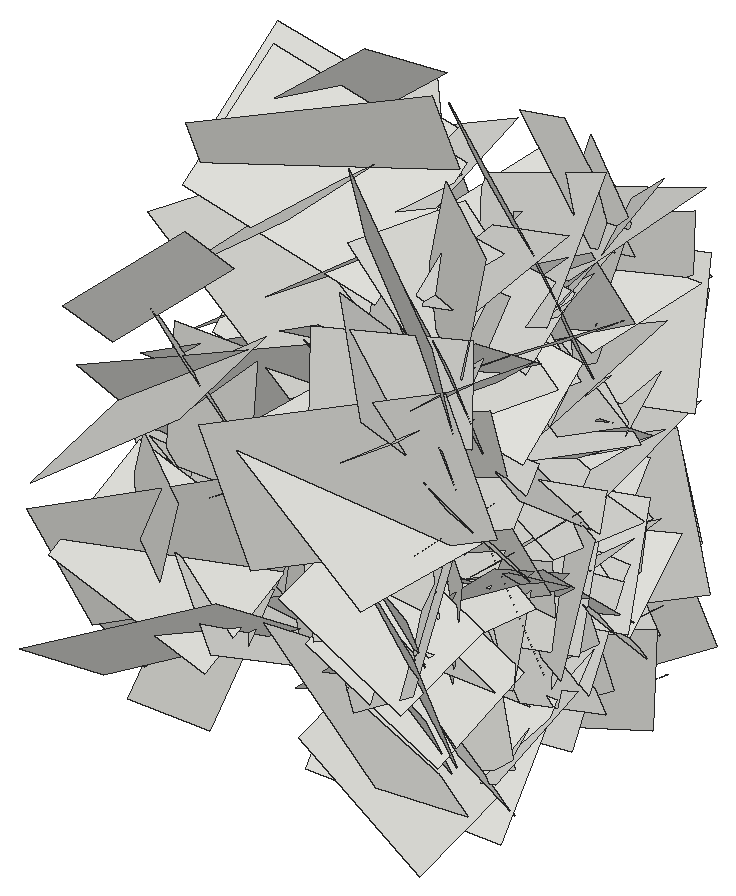
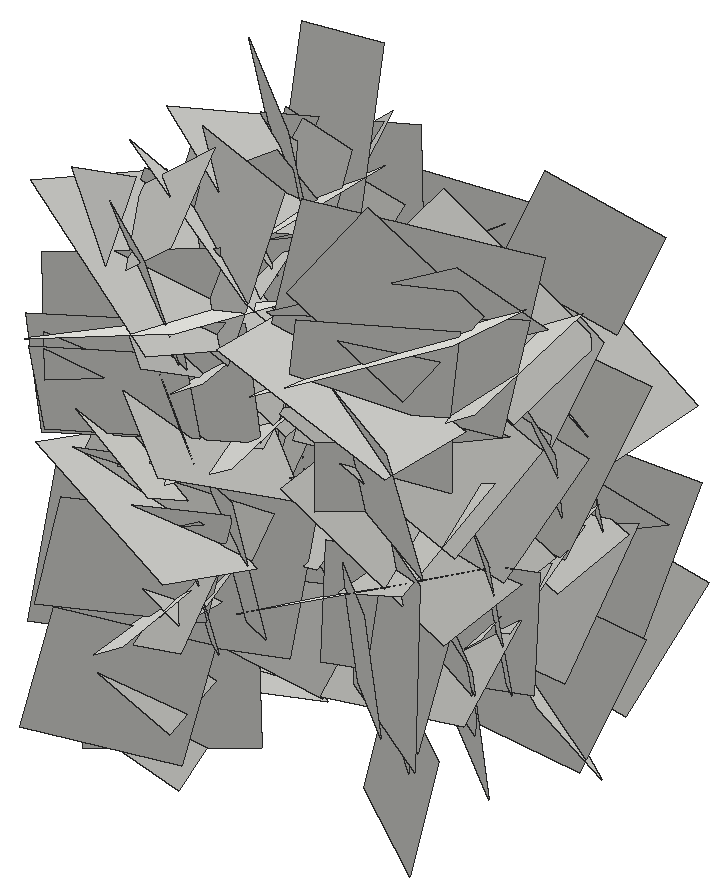
# SketchUp Ruby script. Lengths in inches.
U = 1.inch
M = Sketchup.active_model
def pt(a) = Geom::Point3d.new(a.map { |v| v * U })
def face(e, loops, mat)
  f = e.add_face(loops[0].map { |a| pt(a) })
  loops[1..].each { |l| e.add_face(l.map { |a| pt(a) }).erase! }
  f.material = f.back_material = mat if mat
  f
end
# faces: each face lists its corners as indices into pts; further lists are holes
def faces(e, pts, list, mat = nil) = list.each { |f| face(e, (f[0].is_a?(Array) ? f : [f]).map { |l| l.map { |i| pts[i] } }, mat) }
# xy, xz, yz: faces in a plane at the given z, y or x. An outline is a flat list of corners, or four numbers for a rectangle; further outlines are holes
def ring(l) = l.size == 4 ? [[l[0], l[1]], [l[2], l[1]], [l[2], l[3]], [l[0], l[3]]] : l.each_slice(2).to_a
def flat(e, list, mat, &to3) = list.each { |f| face(e, (f[0].is_a?(Array) ? f : [f]).map { |l| ring(l).map { |u, v| to3.(u, v) } }, mat) }
def xy(e, z, list, mat = nil) = flat(e, list, mat) { |x, y| [x, y, z] }
def xz(e, y, list, mat = nil) = flat(e, list, mat) { |x, z| [x, y, z] }
def yz(e, x, list, mat = nil) = flat(e, list, mat) { |y, z| [x, y, z] }
def lines(e, pts, list) = list.each { |a, b| e.add_line(pt(pts[a]), pt(pts[b])) }
# prism: a flat outline (further loops are holes) pulled along v
def prism(e, loops, v, mat = nil)
  f = face(e, loops, mat); d = Geom::Vector3d.new(v.map { |x| x * U })
  f.pushpull(f.normal.samedirection?(d) ? d.length : -d.length)
end
def box(e, o, s, mat = nil) = prism(e, [[o, [o[0] + s[0], o[1], o[2]], [o[0] + s[0], o[1] + s[1], o[2]], [o[0], o[1] + s[1], o[2]]]], [0, 0, s[2]], mat)
def at(x, y, z, deg = 0) = Geom::Transformation.translation(pt([x, y, z])) * Geom::Transformation.rotation(ORIGIN, Z_AXIS, deg.degrees)
def axes(o, x, y, z) = Geom::Transformation.new([*x, 0, *y, 0, *z, 0, *pt(o).to_a, 1])
def part(name) = M.definitions.add(name)
# library, detail: a bought-in or finely detailed component or shape, given as its bounding box
def library(name, o, s) = part(name).tap { |d| box(d.entities, o, s) }
def detail(e, o, s) = box(e.add_group.entities, o, s)
def put(e, d, t, mat = nil) = e.add_instance(d, t).tap { |i| i.material = mat if mat }
def group(e, t, mat = nil) = e.add_group.tap { |g| g.transformation = t; g.material = mat if mat }.entities
root = M.entities
c1 = part("Component\#6")
p = [[0.01,0,0],[0,3.24,4.54],[4.32,3.24,4.54],[4.33,0,0]]
faces(c1.entities,p,[[0,1,2,3]])
put(root,c1,axes([414.68,149.09,36.34],[0.1737,0.35213,-1.24285],[-0.08,-1.24806,-0.36356],[-1.36694,0.11779,-0.13666]))
put(root,c1,axes([400.91,150.86,30.47],[0.14962,-1.13409,-0.09371],[-0.03493,-0.09847,1.14197],[1.20573,0.13788,0.04471]))
put(root,c1,axes([414.68,150.86,30.47],[-0.14962,-1.13409,-0.09371],[0.03493,-0.09847,1.14197],[-1.20573,0.13788,0.04471]))
put(root,c1,axes([414.68,150.98,27.43],[-0.11329,-0.77541,-0.3635],[0.07754,-0.37325,0.77469],[-0.90445,0.06513,0.11195]))
put(root,c1,axes([410.71,147.9,27.03],[-0.12769,0.03013,0.63893],[-0.01482,0.64988,-0.03329],[0.67785,0.01989,0.11963]))
put(root,c1,axes([404.88,147.9,27.03],[0.12769,0.03013,0.63893],[0.01482,0.64988,-0.03329],[-0.67785,0.01989,0.11963]))
put(root,c1,axes([404.88,149.08,38.35],[-0.0057,0.54335,-0.52891],[0.23788,-0.50408,-0.52014],[-0.76776,-0.16022,-0.15723]))
put(root,c1,axes([410.71,149.08,38.35],[0.0057,0.54335,-0.52891],[-0.23788,-0.50408,-0.52014],[0.76776,-0.16022,-0.15723]))
put(root,c1,axes([400.91,150.2,21.48],[0.03659,-0.96074,0.6365],[0.08804,0.6372,0.9573],[1.21843,-0.01719,-0.08829]))
put(root,c1,axes([414.68,150.2,21.48],[-0.03659,-0.96074,0.6365],[-0.08804,0.6372,0.9573],[-1.21843,-0.01719,-0.08829]))
put(root,c1,axes([414.68,150.44,37.52],[0.01758,-0.03984,-0.83316],[-0.08726,-0.82933,0.03802],[-0.87984,0.08145,-0.02042]))
put(root,c1,axes([410.71,150.81,32.67],[-0.03105,-0.70657,0.01303],[0.00041,0.01303,0.70717],[0.74909,-0.02929,0.00015]))
put(root,c1,axes([410.71,149.71,29.1],[0.04042,0.22115,-0.567],[0.10046,-0.56334,-0.21335],[0.63725,0.07479,0.0696]))
put(root,c1,axes([410.71,147.16,24.1],[-0.03025,0.92414,0.23442],[-0.23339,0.2218,-0.90118],[0.98329,0.08108,-0.20669]))
put(root,c1,axes([410.71,149.63,26.39],[-0.05575,0.3601,-0.58557],[0.15834,-0.56726,-0.36226],[0.71127,0.15451,0.03475]))
put(root,c1,axes([400.91,147.58,26.68],[0.22766,0.71104,0.67114],[-0.02672,0.69094,-0.72395],[1.03608,-0.13842,-0.16614]))
put(root,c1,axes([414.68,147.58,26.68],[-0.22766,0.71104,0.67114],[0.02672,0.69094,-0.72395],[-1.03608,-0.13842,-0.16614]))
put(root,c1,axes([400.91,149.67,23.37],[-0.09539,-0.59855,1.14231],[0.08783,1.14003,0.60389],[1.36418,-0.11525,0.041]))
put(root,c1,axes([414.68,149.67,23.37],[0.09539,-0.59855,1.14231],[-0.08783,1.14003,0.60389],[-1.36418,-0.11525,0.041]))
put(root,c1,axes([414.68,149.65,34.23],[0.2234,-0.54463,1.08834],[0.02633,1.10624,0.54877],[-1.28976,-0.07175,0.19972]))
put(root,c1,axes([410.71,151.89,27.92],[0.07457,-0.37507,-0.49968],[-0.035,-0.50437,0.37394],[0.66135,0.0156,0.07613]))
put(root,c1,axes([414.68,152.86,25.21],[-0.07237,-0.84668,-0.40971],[0.16913,-0.41526,0.83156],[-0.98259,-0.00911,0.17331]))
put(root,c1,axes([410.71,153.18,27.99],[-0.08911,-1.01671,-0.11332],[-0.1646,-0.0997,1.00972],[1.07181,-0.09984,0.14565]))
put(root,c1,axes([414.68,150.4,30.92],[-0.04252,-0.27759,0.76161],[-0.13298,0.75548,0.26875],[-0.84891,-0.10444,-0.08025]))
put(root,c1,axes([400.91,151.25,34.8],[0.16779,0.3958,-0.75565],[0.05631,-0.77163,-0.39305],[0.90246,-0.02545,0.16502]))
put(root,c1,axes([414.68,151.25,34.8],[-0.16779,0.3958,-0.75565],[-0.05631,-0.77163,-0.39305],[-0.90246,-0.02545,0.16502]))
put(root,c1,axes([410.71,152.86,32.22],[-0.07765,-0.95123,0.12327],[-0.10469,0.13045,0.94796],[1.01133,-0.05954,0.1076]))
put(root,c1,axes([414.68,150.92,33.45],[0.01124,-0.40239,0.85237],[-0.02564,0.85203,0.40253],[-0.99881,-0.0264,-0.00074]))
put(root,c1,axes([414.68,150.56,37.37],[-0.01495,0.72639,-0.4873],[-0.06872,-0.48689,-0.7239],[-0.92463,0.02444,0.06168]))
put(root,c1,axes([410.71,150.69,21.46],[-0.08617,-0.06424,0.73191],[0.1147,0.7273,0.07585],[0.77031,-0.11548,0.07058]))
put(root,c1,axes([400.91,154.4,23.625],[-0.0407,-0.65785,-0.83395],[0.03781,-0.83482,0.65689],[1.12528,0.00426,-0.05223]))
put(root,c1,axes([414.68,154.4,23.625],[0.0407,-0.65785,-0.83395],[-0.03781,-0.83482,0.65689],[-1.12528,0.00426,-0.05223]))
put(root,c1,axes([400.91,153.43,27.14],[0.15407,-0.97446,-0.01303],[0.08051,-0.00181,0.98239],[1.02988,0.14592,-0.07485]))
put(root,c1,axes([414.68,153.43,27.14],[-0.15407,-0.97446,-0.01303],[-0.08051,-0.00181,0.98239],[-1.02988,0.14592,-0.07485]))
put(root,c1,axes([400.91,153.58,31.99],[0.17505,-0.32324,-0.90395],[0.10086,-0.9072,0.34179],[1.0126,0.14624,0.12223]))
put(root,c1,axes([414.68,153.58,31.99],[-0.17505,-0.32324,-0.90395],[-0.10086,-0.9072,0.34179],[-1.0126,0.14624,0.12223]))
put(root,c1,axes([410.71,152.7,33.94],[-0.15183,0.13661,-0.74127],[0.04087,-0.75222,-0.14607],[0.79793,0.06452,-0.13357]))
put(root,c1,axes([410.71,153.52,29.46],[-0.08102,0.00764,-0.81457],[-0.10707,-0.81193,0.00187],[0.85682,-0.10074,-0.07679]))
put(root,c1,axes([400.91,152.42,20.54],[-0.05004,-0.6691,0.77955],[0.05919,0.77755,0.67076],[1.08735,-0.07312,-0.00064]))
put(root,c1,axes([414.68,152.42,20.54],[0.05004,-0.6691,0.77955],[-0.05919,0.77755,0.67076],[-1.08735,-0.07312,-0.00064]))
put(root,c1,axes([410.71,154.14,39.875],[-0.07687,-0.17009,-0.90128],[-0.07958,-0.89996,0.17589],[0.96896,-0.0874,-0.05706]))
put(root,c1,axes([414.68,152.27,30.34],[-0.04267,0.47891,-0.74389],[-0.05776,-0.74459,-0.47642],[-0.93603,0.02411,0.06331]))
put(root,c1,axes([400.91,153.125,28.17],[-0.03085,-0.9293,0.97672],[0.26234,0.95667,0.91759],[1.40479,-0.19906,-0.14991]))
put(root,c1,axes([414.68,153.125,28.17],[0.03085,-0.9293,0.97672],[-0.26234,0.95667,0.91759],[-1.40479,-0.19906,-0.14991]))
put(root,c1,axes([400.91,153.14,23.91],[0.18,-1.08552,0.79109],[0.08355,0.80406,1.08641],[1.42134,0.0902,-0.16405]))
put(root,c1,axes([414.68,153.14,23.91],[-0.18,-1.08552,0.79109],[-0.08355,0.80406,1.08641],[-1.42134,0.0902,-0.16405]))
put(root,c1,axes([400.91,151.45,29.33],[0.11063,1.17252,-0.59491],[-0.28501,-0.56514,-1.16101],[1.36425,-0.21315,-0.19431]))
put(root,c1,axes([414.68,151.45,29.33],[-0.11063,1.17252,-0.59491],[0.28501,-0.56514,-1.16101],[-1.36425,-0.21315,-0.19431]))
put(root,c1,axes([410.71,155.3,36.05],[-0.02231,-0.46484,-0.62566],[-0.10069,-0.6197,0.4636],[0.82005,-0.08874,0.0399]))
put(root,c1,axes([400.91,152.14,28.92],[0.00837,0.82237,-0.50147],[0.16225,-0.49618,-0.8113],[1.00803,0.07304,0.13474]))
put(root,c1,axes([414.68,152.14,28.92],[-0.00837,0.82237,-0.50147],[-0.16225,-0.49618,-0.8113],[-1.00803,0.07304,0.13474]))
put(root,c1,axes([414.68,155.63,34.51],[0.04715,-0.7148,-0.47013],[-0.06325,-0.47221,0.71232],[-0.90467,-0.00424,-0.0743]))
put(root,c1,axes([414.68,151.43,29.49],[0.01376,0.93036,0.01045],[0.09599,0.00914,-0.92605],[-0.98156,0.01394,-0.09041]))
put(root,c1,axes([400.91,155.57,33.875],[0.13701,-1.11756,0.11199],[-0.07264,0.10468,1.12363],[1.18833,0.13525,0.05577]))
put(root,c1,axes([414.68,155.57,33.875],[-0.13701,-1.11756,0.11199],[0.07264,0.10468,1.12363],[-1.18833,0.13525,0.05577]))
put(root,c1,axes([410.71,156.34,37.48],[-0.20366,-0.78098,-0.33642],[0.07649,-0.35863,0.79133],[0.89812,-0.14656,-0.14368]))
put(root,c1,axes([414.68,152.31,24.83],[-0.14132,0.38772,0.61473],[-0.11706,0.60692,-0.40674],[-0.76145,-0.16526,-0.05156]))
put(root,c1,axes([410.71,152.23,36.27],[0.17612,0.33723,0.58016],[-0.03508,0.60107,-0.33991],[0.71045,-0.05392,-0.16061]))
put(root,c1,axes([414.68,151.53,22],[0.08087,0.78957,0.40941],[-0.10212,0.41583,-0.78401],[-0.93722,0.02282,0.12075]))
put(root,c1,axes([400.91,156.79,29.67],[0.01777,-0.29003,-1.18393],[-0.05362,-1.18318,0.28913],[1.29096,-0.04516,0.0283]))
put(root,c1,axes([414.68,156.79,29.67],[-0.01777,-0.29003,-1.18393],[0.05362,-1.18318,0.28913],[-1.29096,-0.04516,0.0283]))
put(root,c1,axes([410.71,153.82,25.23],[0.04726,-0.11023,0.59197],[0.093,0.58845,0.10297],[0.63147,-0.07841,-0.05947]))
put(root,c1,axes([410.71,156.05,22.34],[0.04217,-0.56806,-0.37659],[0.07293,-0.37196,0.56834],[0.71876,0.07107,-0.03557]))
put(root,c1,axes([414.68,153.79,24.7],[0.00565,-0.43188,0.90191],[0.04751,0.90112,0.43124],[-1.05892,0.03812,0.02416]))
put(root,c1,axes([400.91,152.25,36.24],[-0.0137,1.21221,-0.26433],[0.01965,-0.26413,-1.21218],[1.31499,0.01657,0.01536]))
put(root,c1,axes([414.68,152.25,36.24],[0.0137,1.21221,-0.26433],[-0.01965,-0.26413,-1.21218],[-1.31499,0.01657,0.01536]))
put(root,c1,axes([400.91,157.5625,26.25],[0.15158,-0.38022,-1.22414],[-0.0526,-1.23246,0.37701],[1.35773,-0.0053,0.15127]))
put(root,c1,axes([414.68,157.5625,26.25],[-0.15158,-0.38022,-1.22414],[0.0526,-1.23246,0.37701],[-1.35773,-0.0053,0.15127]))
put(root,c1,axes([400.91,156.02,28.65],[-0.0619,-0.85924,0.62732],[0.17366,0.61351,0.85557],[1.11425,-0.14335,-0.09849]))
put(root,c1,axes([414.68,156.02,28.65],[0.0619,-0.85924,0.62732],[-0.17366,0.61351,0.85557],[-1.11425,-0.14335,-0.09849]))
put(root,c1,axes([400.91,153.73,28.3],[-0.01858,0.99462,-0.84655],[0.29457,-0.8244,-0.97435],[1.35277,0.19318,0.20054]))
put(root,c1,axes([414.68,153.73,28.3],[0.01858,0.99462,-0.84655],[-0.29457,-0.8244,-0.97435],[-1.35277,0.19318,0.20054]))
put(root,c1,axes([410.71,153.92,21.15],[-0.0271,-0.2919,0.8704],[-0.20523,0.85287,0.28034],[0.95124,0.17569,0.08528]))
put(root,c1,axes([404.88,157.4,31.875],[0.05779,-0.51798,-0.36432],[0.0587,-0.36037,0.52065],[-0.6687,-0.0764,0.01422]))
put(root,c1,axes([410.71,157.4,31.875],[-0.05779,-0.51798,-0.36432],[-0.0587,-0.36037,0.52065],[0.6687,-0.0764,0.01422]))
put(root,c1,axes([414.68,156.72,22.08],[0.00521,-0.94479,0.50901],[0.17637,0.50353,0.93301],[-1.12382,0.07464,0.14878]))
put(root,c1,axes([414.68,155.99,38.05],[-0.0315,0.52335,-0.79271],[0.01447,-0.79278,-0.52391],[-1.00678,-0.02777,0.01727]))
put(root,c1,axes([400.91,157.84,26.69],[0.16666,-0.37984,-0.88441],[0.10341,-0.88523,0.39754],[1.01503,0.15255,0.10471]))
put(root,c1,axes([414.68,157.84,26.69],[-0.16666,-0.37984,-0.88441],[-0.10341,-0.88523,0.39754],[-1.01503,0.15255,0.10471]))
put(root,c1,axes([414.68,157.73,31.39],[0.13129,-0.92283,0.37392],[-0.04334,0.37177,0.93107],[-1.05456,-0.13017,0.00829]))
put(root,c1,axes([400.91,154.59,24.16],[-0.1724,0.15274,1.09758],[0.17194,1.10067,-0.12914],[1.16199,-0.14021,0.18195]))
put(root,c1,axes([414.68,154.59,24.16],[0.1724,0.15274,1.09758],[-0.17194,1.10067,-0.12914],[-1.16199,-0.14021,0.18195]))
put(root,c1,axes([414.68,154.45,36.57],[-0.07713,0.81709,0.22722],[-0.03645,0.22503,-0.82021],[-0.89825,-0.07929,0.01378]))
put(root,c1,axes([414.68,158.82,28.52],[0.0834,-0.34729,-0.88838],[-0.00654,-0.89156,0.34799],[-1.01106,-0.02288,-0.07553]))
put(root,c1,axes([400.91,158.93,27.77],[-0.0679,-1.16178,0.21088],[0.08573,0.20637,1.16154],[1.24867,-0.07734,-0.06828]))
put(root,c1,axes([414.68,158.93,27.77],[0.0679,-1.16178,0.21088],[-0.08573,0.20637,1.16154],[-1.24867,-0.07734,-0.06828]))
put(root,c1,axes([400.91,153.92,36.42],[0.14295,0.82362,0.79821],[0.11339,0.79118,-0.83443],[1.21047,-0.17138,-0.0161]))
put(root,c1,axes([414.68,153.92,36.42],[-0.14295,0.82362,0.79821],[-0.11339,0.79118,-0.83443],[-1.21047,-0.17138,-0.0161]))
put(root,c1,axes([400.91,158.37,30.5],[0.12568,-1.12455,0.31778],[-0.06348,0.31314,1.13049],[1.23707,0.13032,0.02572]))
put(root,c1,axes([414.68,158.37,30.5],[-0.12568,-1.12455,0.31778],[0.06348,0.31314,1.13049],[-1.23707,0.13032,0.02572]))
put(root,c1,axes([400.91,156.14,33.68],[0.06217,-0.55405,1.15944],[0.03014,1.16092,0.55332],[1.36179,-0.0004,-0.06518]))
put(root,c1,axes([414.68,156.14,33.68],[-0.06217,-0.55405,1.15944],[-0.03014,1.16092,0.55332],[-1.36179,-0.0004,-0.06518]))
put(root,c1,axes([410.71,158.01,30.39],[0.08038,-0.60995,0.00551],[-0.02253,0.00291,0.6143],[0.64618,0.07598,0.02073]))
put(root,c1,axes([414.68,152.65,32.7],[0.31384,1.21799,0.62272],[0.13011,0.61092,-1.25326],[-1.44417,0.31973,0.02242]))
put(root,c1,axes([400.91,156.45,32.24],[0.14884,0.843,-0.57449],[-0.06248,-0.57223,-0.85409],[1.07954,-0.14935,0.02978]))
put(root,c1,axes([414.68,156.45,32.24],[-0.14884,0.843,-0.57449],[0.06248,-0.57223,-0.85409],[-1.07954,-0.14935,0.02978]))
put(root,c1,axes([400.91,158.66,27.8],[0.19419,0.10037,-0.91545],[-0.10975,-0.92523,-0.12216],[0.97001,-0.12478,0.16945]))
put(root,c1,axes([414.68,158.66,27.8],[-0.19419,0.10037,-0.91545],[0.10975,-0.92523,-0.12216],[-0.97001,-0.12478,0.16945]))
put(root,c1,axes([410.71,158.73,27.09],[-0.13155,-0.14233,-0.74779],[-0.00006,-0.75766,0.14422],[0.80689,-0.02326,-0.12191]))
put(root,c1,axes([414.68,156.02,27.27],[-0.01737,0.78195,0.05447],[-0.0729,0.05284,-0.77921],[-0.82768,-0.02106,0.06749]))
put(root,c1,axes([400.91,159.15,23.91],[0.14407,0.13595,-0.90237],[-0.02833,-0.91134,-0.14133],[0.9669,-0.04696,0.13032]))
put(root,c1,axes([414.68,159.15,23.91],[-0.14407,0.13595,-0.90237],[0.02833,-0.91134,-0.14133],[-0.9669,-0.04696,0.13032]))
put(root,c1,axes([410.71,156.49,28.09],[0.01227,0.36562,0.53928],[0.0952,0.53332,-0.36351],[0.68404,-0.08079,0.04092]))
put(root,c1,axes([404.88,156.65,23.33],[-0.01341,0.01203,0.69899],[0.10657,0.69187,-0.01009],[-0.73333,0.10033,-0.01425]))
put(root,c1,axes([410.71,156.65,23.33],[0.01341,0.01203,0.69899],[-0.10657,0.69187,-0.01009],[0.73333,0.10033,-0.01425]))
put(root,c1,axes([414.68,158.65,23.12],[0.03,-0.65446,0.65644],[-0.11713,0.64968,0.65248],[-0.97555,-0.09812,-0.05816]))
put(root,c1,axes([414.68,160.05,30.35],[0.12426,0.20575,-1.35522],[0.11745,-1.35714,-0.19646],[-1.44825,-0.0924,-0.13221]))
put(root,c1,axes([400.91,160.05,30.35],[-0.12426,0.20575,-1.35522],[-0.11745,-1.35714,-0.19646],[1.44825,-0.0924,-0.13221]))
put(root,c1,axes([414.68,154.61,36.92],[0.07328,1.03426,0.55463],[0.26621,0.52968,-1.01904],[-1.21518,0.17841,-0.1898]))
put(root,c1,axes([414.68,160.42,26.72],[0.04031,-0.6417,-0.5437],[-0.04231,-0.54502,0.64047],[-0.89052,-0.00315,-0.05504]))
put(root,c1,axes([404.88,160.09,33.87],[0.13785,-0.16653,-0.67513],[0.04892,-0.68326,0.17743],[-0.73546,-0.07666,-0.11474]))
put(root,c1,axes([410.71,160.09,33.87],[-0.13785,-0.16653,-0.67513],[-0.04892,-0.68326,0.17743],[0.73546,-0.07666,-0.11474]))
put(root,c1,axes([400.91,154.96,37.56],[-0.27688,1.1515,0.31839],[0.11464,0.34737,-1.16756],[1.26119,0.22122,0.17603]))
put(root,c1,axes([414.68,154.96,37.56],[0.27688,1.1515,0.31839],[-0.11464,0.34737,-1.16756],[-1.26119,0.22122,0.17603]))
put(root,c1,axes([410.71,159.35,19.53],[0.12506,-0.65018,0.20227],[-0.00025,0.20525,0.65988],[0.72178,0.11273,-0.03482]))
put(root,c1,axes([404.88,157.59,40.82],[0.16311,0.68993,-0.43022],[0.09586,-0.44966,-0.68876],[-0.85651,0.08106,-0.15901]))
put(root,c1,axes([410.71,157.59,40.82],[-0.16311,0.68993,-0.43022],[-0.09586,-0.44966,-0.68876],[0.85651,0.08106,-0.15901]))
put(root,c1,axes([410.71,159.76,21.63],[0.09665,-0.666,0.12875],[-0.03078,0.12595,0.67212],[0.71837,0.095,0.01147]))
put(root,c1,axes([404.88,161,38.46],[0.19651,-0.13504,-0.81499],[0.03185,-0.8336,0.14496],[-0.87508,-0.06067,-0.17773]))
put(root,c1,axes([410.71,161,38.46],[-0.19651,-0.13504,-0.81499],[-0.03185,-0.8336,0.14496],[0.87508,-0.06067,-0.17773]))
put(root,c1,axes([400.91,156.69,29.48],[-0.02364,1.01192,0.31394],[0.16386,0.31376,-1.00035],[1.11105,-0.02474,0.15421]))
put(root,c1,axes([414.68,156.69,29.48],[0.02364,1.01192,0.31394],[-0.16386,0.31376,-1.00035],[-1.11105,-0.02474,0.15421]))
put(root,c1,axes([410.71,158.75,26.14],[0.12859,0.59437,-0.23179],[-0.06253,-0.22448,-0.60651],[0.67335,-0.13435,-0.01206]))
put(root,c1,axes([410.71,160.84,30.26],[0.09118,-0.56201,-0.30691],[0.0596,-0.30185,0.56849],[0.67615,0.1024,-0.00872]))
put(root,c1,axes([414.68,160.9375,37.33],[-0.13153,0.12633,-0.90974],[0.10231,-0.91113,-0.13969],[-0.96819,-0.11344,0.10882]))
put(root,c1,axes([400.91,161.68,35.57],[-0.09547,-0.29138,-1.10436],[0.14499,-1.10257,0.27976],[1.20197,0.10985,-0.12146]))
put(root,c1,axes([414.68,161.68,35.57],[0.09547,-0.29138,-1.10436],[-0.14499,-1.10257,0.27976],[-1.20197,0.10985,-0.12146]))
put(root,c1,axes([400.91,161.74,34.71],[0.1652,-1.10091,-0.16395],[0.26327,-0.12698,1.08875],[1.15009,0.1872,-0.22568]))
put(root,c1,axes([414.68,161.74,34.71],[-0.1652,-1.10091,-0.16395],[-0.26327,-0.12698,1.08875],[-1.15009,0.1872,-0.22568]))
put(root,c1,axes([404.88,158.03,24.73],[0.19324,-0.05037,0.89121],[0.15909,0.89838,0.02008],[-0.93272,0.1428,0.18806]))
put(root,c1,axes([410.71,158.03,24.73],[-0.19324,-0.05037,0.89121],[-0.15909,0.89838,0.02008],[0.93272,0.1428,0.18806]))
put(root,c1,axes([410.71,159.1875,20.3125],[-0.01409,-0.35632,0.80543],[-0.16766,0.79339,0.34838],[0.91839,0.13938,0.07596]))
put(root,c1,axes([414.68,161.57,34.4],[0.05292,-0.24359,-0.78611],[-0.1523,-0.77804,0.23197],[-0.85897,0.12294,-0.08956]))
